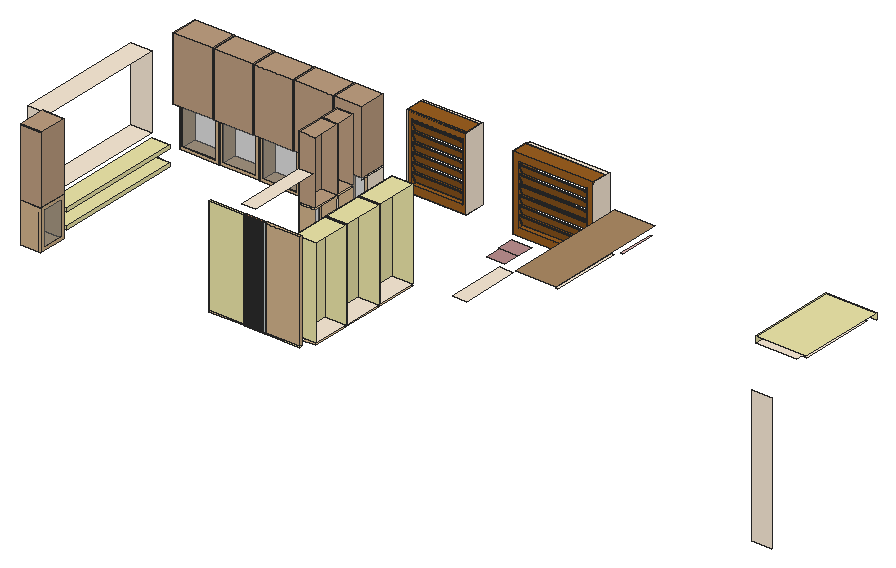
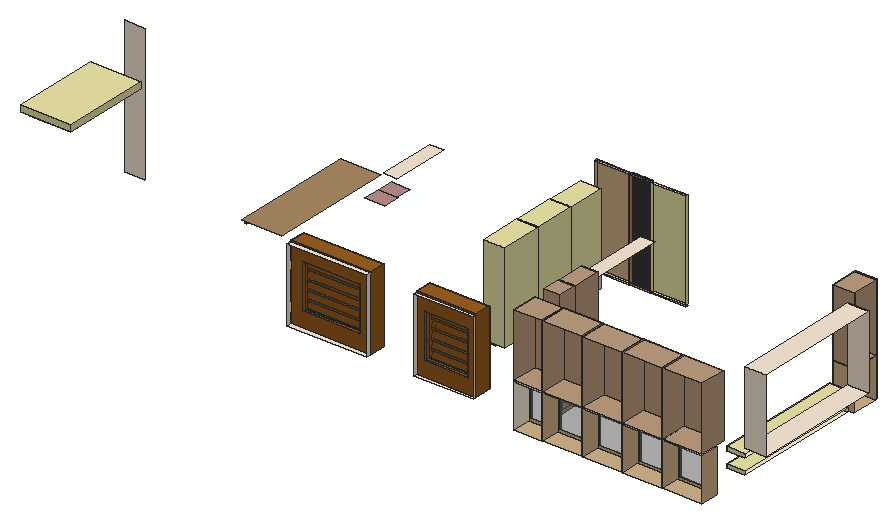
# SketchUp Ruby script. Lengths in inches.
U = 1.inch
M = Sketchup.active_model
def pt(a) = Geom::Point3d.new(a.map { |v| v * U })
def face(e, loops, mat)
  f = e.add_face(loops[0].map { |a| pt(a) })
  loops[1..].each { |l| e.add_face(l.map { |a| pt(a) }).erase! }
  f.material = f.back_material = mat if mat
  f
end
# faces: each face lists its corners as indices into pts; further lists are holes
def faces(e, pts, list, mat = nil) = list.each { |f| face(e, (f[0].is_a?(Array) ? f : [f]).map { |l| l.map { |i| pts[i] } }, mat) }
# xy, xz, yz: faces in a plane at the given z, y or x. An outline is a flat list of corners, or four numbers for a rectangle; further outlines are holes
def ring(l) = l.size == 4 ? [[l[0], l[1]], [l[2], l[1]], [l[2], l[3]], [l[0], l[3]]] : l.each_slice(2).to_a
def flat(e, list, mat, &to3) = list.each { |f| face(e, (f[0].is_a?(Array) ? f : [f]).map { |l| ring(l).map { |u, v| to3.(u, v) } }, mat) }
def xy(e, z, list, mat = nil) = flat(e, list, mat) { |x, y| [x, y, z] }
def xz(e, y, list, mat = nil) = flat(e, list, mat) { |x, z| [x, y, z] }
def yz(e, x, list, mat = nil) = flat(e, list, mat) { |y, z| [x, y, z] }
def lines(e, pts, list) = list.each { |a, b| e.add_line(pt(pts[a]), pt(pts[b])) }
# prism: a flat outline (further loops are holes) pulled along v
def prism(e, loops, v, mat = nil)
  f = face(e, loops, mat); d = Geom::Vector3d.new(v.map { |x| x * U })
  f.pushpull(f.normal.samedirection?(d) ? d.length : -d.length)
end
def box(e, o, s, mat = nil) = prism(e, [[o, [o[0] + s[0], o[1], o[2]], [o[0] + s[0], o[1] + s[1], o[2]], [o[0], o[1] + s[1], o[2]]]], [0, 0, s[2]], mat)
def at(x, y, z, deg = 0) = Geom::Transformation.translation(pt([x, y, z])) * Geom::Transformation.rotation(ORIGIN, Z_AXIS, deg.degrees)
def axes(o, x, y, z) = Geom::Transformation.new([*x, 0, *y, 0, *z, 0, *pt(o).to_a, 1])
def part(name) = M.definitions.add(name)
# library, detail: a bought-in or finely detailed component or shape, given as its bounding box
def library(name, o, s) = part(name).tap { |d| box(d.entities, o, s) }
def detail(e, o, s) = box(e.add_group.entities, o, s)
def put(e, d, t, mat = nil) = e.add_instance(d, t).tap { |i| i.material = mat if mat }
def group(e, t, mat = nil) = e.add_group.tap { |g| g.transformation = t; g.material = mat if mat }.entities
root = M.entities
M.materials.add("Maquette Wood B01 12cm").color = [172, 139, 100]
M.materials.add("Plywood A 50cm\#1").color = [191, 159, 129]
M.materials.add("Wood EXN").color = [155, 95, 32]
M.materials.add("[0028_AntiqueWhite]").color = [250, 235, 215]
M.materials.add("[0035_Tan]").color = [210, 180, 140]
M.materials.add("[0048_PaleGoldenrod]").color = [238, 232, 170]
M.materials.add("[0119_RosyBrown]").color = [188, 143, 143]
M.materials.add("[Textile Leaves Green]").color = [226, 183, 181]
M.materials.add("[Translucent Glass Gray]").color = [128, 128, 128]
M.materials["[Translucent Glass Gray]"].alpha = 0.5
M.materials.add("[Wallpaper Dog Bone]").color = [213, 224, 224]
M.materials.add("[Wood Veneer 02]").color = [190, 128, 91]
c1 = part("Group\#38")
prism(c1.entities,[[[0,1.97,1.57],[0,0.24,0.19],[0,0.22,0.17],[0,0.2,0.14],[0,0.19,0.11],[0,0.2,0.08],[0,0.2,0.05],[0,0.22,0.02],[0,0.24,0],[0,0.27,-0.02],[0,0.3,-0.03],[0,0.34,-0.03],[0,0.37,-0.02],[0,0.39,0],[0,2.36,1.57]]],[-67.04,0,0])
c2 = part("Wood+Window")
g1 = group(c2.entities,at(47.24,0,19.69),"Wood EXN")
g2 = group(g1,at(-47.24,5.91,0))
xy(g2,-19.69,[[0,-5.91,27.56,0]])
xy(g2,-17.72,[[1.97,-3.9375,25.59,0]])
xy(g2,-15.75,[[3.9375,-5.91,23.62,-4.92],[3.9375,-4.92,23.62,-3.9375]])
xy(g2,-3.9375,[[3.9375,-5.91,23.62,-4.92],[3.9375,-4.92,23.62,-3.9375]])
xy(g2,-1.97,[[1.97,-3.9375,25.59,0]])
xy(g2,0,[[0,-5.91,27.56,0]])
xz(g2,-5.91,[[[0,-19.69,27.56,0],[3.9375,-15.75,23.62,-3.9375]]])
xz(g2,-3.9375,[[[1.97,-17.72,25.59,-1.97],[3.9375,-15.75,23.62,-3.9375]]])
xz(g2,0,[[[0,-19.69,27.56,0],[1.97,-17.72,25.59,-1.97]]])
yz(g2,0,[[-5.91,-19.69,0,0]])
yz(g2,1.97,[[-3.9375,-17.72,0,-1.97]])
yz(g2,3.9375,[[-5.91,-15.75,-4.92,-3.9375],[-4.92,-15.75,-3.9375,-3.9375]])
yz(g2,23.62,[[-5.91,-15.75,-4.92,-3.9375],[-4.92,-15.75,-3.9375,-3.9375]])
yz(g2,25.59,[[-3.9375,-17.72,0,-1.97]])
yz(g2,27.56,[[-5.91,-19.69,0,0]])
g3 = group(g1,at(-20.98,5.88,-0.4))
put(g3,c1,axes([-24.3,0,-14.09],[-0.35238,0,0],[0,0,-1.2344],[0,-1,0]))
put(g3,c1,axes([-24.3,0,-11.66],[-0.35238,0,0],[0,0,-1.2344],[0,-1,0]))
put(g3,c1,axes([-24.3,0,-9.23],[-0.35238,0,0],[0,0,-1.2344],[0,-1,0]))
put(g3,c1,axes([-24.3,0,-6.8],[-0.35238,0,0],[0,0,-1.2344],[0,-1,0]))
put(g3,c1,axes([-24.3,0,-4.375],[-0.35238,0,0],[0,0,-1.2344],[0,-1,0]))
put(g3,c1,axes([-24.3,0,-1.94],[-0.35238,0,0],[0,0,-1.2344],[0,-1,0]))
xy(root,67.4375,[[9,365.9375,18.125,377.9375],[86.0625,421,93,433],[86.0625,433.5,93,441.5625],[10,450.9375,27,459],[27.5,450.9375,44.5,459],
  [45,450.9375,62,459],[62.5,450.9375,79.5,459],[80,450.9375,92,459]],"[0035_Tan]")
xy(root,68.47,[[46.04,450.9375,60.96,451.3125]],"[Translucent Glass Gray]")
xy(root,68.57,[[11.13,450.9375,25.87,451.25]],"[Translucent Glass Gray]")
xy(root,68.6,[[17.9375,367.1,18.125,376.78],[28.66,450.9375,43.34,451.25]],"[Translucent Glass Gray]")
xy(root,68.625,[[86.0625,422.1875,86.4375,431.8125]],"[Translucent Glass Gray]")
xy(root,68.67,[[86.0625,434.73,86.25,440.33]],"[Translucent Glass Gray]")
xy(root,68.6875,[[81.25,450.9375,90.75,451.1875]],"[Translucent Glass Gray]")
xy(root,68.7,[[63.76,450.9375,78.24,451.125]],"[Translucent Glass Gray]")
xy(root,69.2,[[9,380.875,16.9375,437.125]],"[0028_AntiqueWhite]")
xy(root,70.71,[[129.3125,369,134.6875,385.5],[129.3125,386,134.6875,403.5],[129.3125,404,134.6875,422]],"[0035_Tan]")
xy(root,70.77,[[9,380.875,16.9375,437.125]],"[0048_PaleGoldenrod]")
xy(root,71.3125,[[125.5625,369.5,134.6875,385.5],[125.5625,386,134.6875,403.5],[125.5625,404,134.6875,422]],"[0028_AntiqueWhite]")
xy(root,72.59,[[94,361.9375,109,363]],"[0035_Tan]")
xy(root,72.59,[[118.6875,361.9375,133.6875,363]],"[0048_PaleGoldenrod]")
xy(root,72.59,[[109.5,361.9375,118.1875,363]],"[Wood Veneer 02]")
xy(root,73.1875,[[109.5,361.5625,109.82,361.9375],[110.02,361.5625,110.35,361.9375],[110.55,361.5625,110.87,361.9375],[111.07,361.5625,111.39,361.9375],[111.59,361.5625,111.92,361.9375],
  [112.12,361.5625,112.44,361.9375],[112.64,361.5625,112.96,361.9375],[113.16,361.5625,113.49,361.9375],[113.6875,361.5625,114.01,361.9375],[114.21,361.5625,114.54,361.9375],
  [114.73,361.5625,115.06,361.9375],[115.26,361.5625,115.58,361.9375],[115.78,361.5625,116.11,361.9375],[116.3,361.5625,116.63,361.9375],[116.83,361.5625,117.15,361.9375],
  [117.35,361.5625,117.68,361.9375],[117.875,361.5625,118.2,361.9375],[109.5,361.9375,118.1875,363]],"[0028_AntiqueWhite]")
xy(root,73.1875,[[118.6875,361.9375,133.6875,363]],"[0035_Tan]")
xy(root,73.1875,[[94,361.9375,109,363]],"[0048_PaleGoldenrod]")
xy(root,76.0625,[[9,380.875,16.9375,437.125]],"[0028_AntiqueWhite]")
xy(root,77.6875,[[9,380.875,16.9375,437.125]],"[0048_PaleGoldenrod]")
xy(root,79.6875,[[0,380.875,9,437.125],[102.5,459,128.4375,468],[148.875,459,183.6875,468]],"[0028_AntiqueWhite]")
xy(root,83.55,[[17.9375,367.1,18.125,376.78]],"[Translucent Glass Gray]")
xy(root,84.71,[[9,365.9375,18.125,377.9375]],"[0035_Tan]")
xy(root,84.86,[[63.76,450.9375,78.24,451.125]],"[Translucent Glass Gray]")
xy(root,84.875,[[81.25,450.9375,90.75,451.1875]],"[Translucent Glass Gray]")
xy(root,84.89,[[86.0625,434.73,86.25,440.33]],"[Translucent Glass Gray]")
xy(root,84.9375,[[86.0625,422.1875,86.4375,431.8125]],"[Translucent Glass Gray]")
xy(root,84.96,[[28.66,450.9375,43.34,451.25]],"[Translucent Glass Gray]")
xy(root,84.99,[[11.13,450.9375,25.87,451.25]],"[Translucent Glass Gray]")
xy(root,85.02,[[9,365.9375,18.125,377.9375]],"Plywood A 50cm\#1")
xy(root,85.09,[[46.04,450.9375,60.96,451.3125]],"[Translucent Glass Gray]")
xy(root,86.125,[[86.0625,421,93,433],[86.0625,433.5,93,441.5625],[10,450.9375,27,459],[27.5,450.9375,44.5,459],[45,450.9375,62,459],
  [62.5,450.9375,79.5,459],[80,450.9375,92,459]],"[0035_Tan]")
xy(root,86.6875,[[86.0625,421,93,433],[86.0625,433.5,93,441.5625],[10,447.5,27,459],[27.5,447.5,44.5,459],[45,447.5,62,459],
  [62.5,447.5,79.5,459],[80,447.5,92,459]],"Plywood A 50cm\#1")
xy(root,103.4,[[212.3125,438.47,213,454.22]],"[Textile Leaves Green]")
xy(root,104.55,[[211.3125,404.13,212.3125,434.43]],"[0028_AntiqueWhite]")
xy(root,106,[[195,402.6875,212.3125,456.8125]],"Maquette Wood B01 12cm")
xy(root,106,[[189,375.81,195,401.3125],[93,381.06,99,412.0625]],"[0028_AntiqueWhite]")
xy(root,106,[[181,404.5,189,411.4375],[180.4375,411.4375,189,418.8125]],"[0119_RosyBrown]")
xy(root,108.8,[[293.125,410.9375,293.125,449.0625,311,449.0625,311,446.36,313.125,446.36,313.125,413.64,311,413.64,311,410.9375]],"[0028_AntiqueWhite]")
xy(root,110.4375,[[125.5625,369.5,134.6875,385.5],[125.5625,386,134.6875,403.5],[125.5625,404,134.6875,422]],"[0048_PaleGoldenrod]")
xy(root,111.5,[[293.125,410.9375,315,449.0625]],"[0048_PaleGoldenrod]")
xy(root,111.66,[[0,380.875,9,437.125],[102.5,459,128.4375,468],[148.875,459,183.6875,468]],"[0028_AntiqueWhite]")
xy(root,114.3125,[[9,365.9375,18.125,377.9375],[86.0625,421,93,433],[86.0625,433.5,93,441.5625],[10,447.5,27,459],[27.5,447.5,44.5,459],
  [45,447.5,62,459],[62.5,447.5,79.5,459],[80,447.5,92,459]],"Plywood A 50cm\#1")
xy(root,115.7,[[118.6875,361.9375,133.6875,363]],"[0035_Tan]")
xy(root,115.7,[[94,361.9375,109,363]],"[0048_PaleGoldenrod]")
xy(root,115.7,[[109.5,361.5625,109.82,361.9375],[110.02,361.5625,110.35,361.9375],[110.55,361.5625,110.87,361.9375],[111.07,361.5625,111.39,361.9375],[111.59,361.5625,111.92,361.9375],
  [112.12,361.5625,112.44,361.9375],[112.64,361.5625,112.96,361.9375],[113.16,361.5625,113.49,361.9375],[113.6875,361.5625,114.01,361.9375],[114.21,361.5625,114.54,361.9375],
  [114.73,361.5625,115.06,361.9375],[115.26,361.5625,115.58,361.9375],[115.78,361.5625,116.11,361.9375],[116.3,361.5625,116.63,361.9375],[116.83,361.5625,117.15,361.9375],
  [117.35,361.5625,117.68,361.9375],[117.875,361.5625,118.2,361.9375]],"[Wallpaper Dog Bone]")
xy(root,115.7,[[109.5,361.9375,118.1875,363]],"[Wood Veneer 02]")
xz(root,361.9375,[[109.5,73.1875,109.82,115.7],[110.02,73.1875,110.35,115.7],[110.55,73.1875,110.87,115.7],[111.07,73.1875,111.39,115.7],[111.59,73.1875,111.92,115.7],
  [112.12,73.1875,112.44,115.7],[112.64,73.1875,112.96,115.7],[113.16,73.1875,113.49,115.7],[113.6875,73.1875,114.01,115.7],[114.21,73.1875,114.54,115.7],
  [114.73,73.1875,115.06,115.7],[115.26,73.1875,115.58,115.7],[115.78,73.1875,116.11,115.7],[116.3,73.1875,116.63,115.7],[116.83,73.1875,117.15,115.7],
  [117.35,73.1875,117.68,115.7],[117.875,73.1875,118.1875,115.7]],"[0028_AntiqueWhite]")
xz(root,361.9375,[[118.6875,73.1875,133.6875,115.7]],"[0035_Tan]")
xz(root,361.9375,[[94,73.1875,109,115.7]],"[0048_PaleGoldenrod]")
xz(root,361.9375,[[109.82,73.1875,110.02,115.7],[110.35,73.1875,110.55,115.7],[110.87,73.1875,111.07,115.7],[111.39,73.1875,111.59,115.7],[111.92,73.1875,112.12,115.7],
  [112.44,73.1875,112.64,115.7],[112.96,73.1875,113.16,115.7],[113.49,73.1875,113.6875,115.7],[114.01,73.1875,114.21,115.7],[114.54,73.1875,114.73,115.7],
  [115.06,73.1875,115.26,115.7],[115.58,73.1875,115.78,115.7],[116.11,73.1875,116.3,115.7],[116.63,73.1875,116.83,115.7],[117.15,73.1875,117.35,115.7],
  [117.68,73.1875,117.875,115.7]],"[Wood Veneer 02]")
xz(root,364.16,[[17.9375,68.72,18.125,83.43]],"[Translucent Glass Gray]")
xz(root,365.4375,[[9,85.02,18.125,114.3125]],"Plywood A 50cm\#1")
xz(root,365.4375,[[9,67.4375,18.125,84.71]],"[0035_Tan]")
xz(root,365.9375,[[9,85.02,18.125,114.3125]],"Plywood A 50cm\#1")
xz(root,365.9375,[[9,67.4375,18.125,84.71]],"[0035_Tan]")
xz(root,367.1,[[17.9375,68.6,18.125,83.55]],"[0028_AntiqueWhite]")
xz(root,369.5,[[125.5625,71.3125,134.6875,110.4375]],"[0048_PaleGoldenrod]")
xz(root,376.78,[[17.9375,68.6,18.125,83.55]],"[0028_AntiqueWhite]")
xz(root,377.9375,[[9,85.02,18.125,114.3125]],"Plywood A 50cm\#1")
xz(root,377.9375,[[9,67.4375,18.125,84.71]],"[0035_Tan]")
xz(root,380.875,[[0,79.6875,9,111.66]],"[0028_AntiqueWhite]")
xz(root,380.875,[[9,69.2,16.9375,70.77],[9,76.0625,16.9375,77.6875]],"[0048_PaleGoldenrod]")
xz(root,381.0625,[[315,52.5,324,111.5]],"[0028_AntiqueWhite]")
xz(root,385.5,[[125.5625,71.3125,134.6875,110.4375]],"[0048_PaleGoldenrod]")
xz(root,386,[[125.5625,71.3125,134.6875,110.4375]],"[0048_PaleGoldenrod]")
xz(root,403.5,[[125.5625,71.3125,134.6875,110.4375]],"[0048_PaleGoldenrod]")
xz(root,404,[[125.5625,71.3125,134.6875,110.4375]],"[0048_PaleGoldenrod]")
xz(root,421,[[86.0625,86.6875,93,114.3125]],"Plywood A 50cm\#1")
xz(root,421,[[86.0625,67.4375,93,86.125]],"[0035_Tan]")
xz(root,422,[[125.5625,71.3125,134.6875,110.4375]],"[0048_PaleGoldenrod]")
xz(root,422.1875,[[86.0625,68.625,86.4375,84.9375]],"[Translucent Glass Gray]")
xz(root,431.8125,[[86.0625,68.625,86.4375,84.9375]],"[Translucent Glass Gray]")
xz(root,433,[[86.0625,86.6875,93,114.3125]],"Plywood A 50cm\#1")
xz(root,433,[[86.0625,67.4375,93,86.125]],"[0035_Tan]")
xz(root,433.5,[[86.0625,86.6875,93,114.3125]],"Plywood A 50cm\#1")
xz(root,433.5,[[86.0625,67.4375,93,86.125]],"[0035_Tan]")
xz(root,434.73,[[86.0625,68.67,86.25,84.89]],"[Translucent Glass Gray]")
xz(root,437.125,[[0,79.6875,9,111.66]],"[0028_AntiqueWhite]")
xz(root,437.125,[[9,69.2,16.9375,70.77],[9,76.0625,16.9375,77.6875]],"[0048_PaleGoldenrod]")
xz(root,440.33,[[86.0625,68.67,86.25,84.89]],"[Translucent Glass Gray]")
xz(root,441.5625,[[86.0625,86.6875,93,114.3125]],"Plywood A 50cm\#1")
xz(root,441.5625,[[86.0625,67.4375,93,86.125]],"[0035_Tan]")
xz(root,447.5,[[10,86.6875,27,114.3125],[27.5,86.6875,44.5,114.3125],[45,86.6875,62,114.3125],[62.5,86.6875,79.5,114.3125],[80,86.6875,92,114.3125]],"Plywood A 50cm\#1")
xz(root,449.0625,[[293.125,108.8,315,111.5]],"[0048_PaleGoldenrod]")
xz(root,450.9375,[[[10,67.4375,27,86.125],[11.13,68.57,25.87,84.99]],[[27.5,67.4375,44.5,86.125],[28.66,68.6,43.34,84.96]],[[45,67.4375,62,86.125],[46.04,68.47,60.96,85.09]],[[62.5,67.4375,79.5,86.125],[63.76,68.7,78.24,84.86]],[[80,67.4375,92,86.125],[81.25,68.6875,90.75,84.875]]],"[0035_Tan]")
xz(root,451.125,[[63.76,68.7,78.24,84.86]],"[Translucent Glass Gray]")
xz(root,451.1875,[[81.25,68.6875,90.75,84.875]],"[Translucent Glass Gray]")
xz(root,451.25,[[11.13,68.57,25.87,84.99],[28.66,68.6,43.34,84.96]],"[Translucent Glass Gray]")
xz(root,451.3125,[[46.04,68.47,60.96,85.09]],"[Translucent Glass Gray]")
xz(root,459,[[27,67.4375,27.5,84.6875],[44.5,67.4375,45,84.6875],[62,67.4375,62.5,84.6875],[79.5,67.4375,80,84.6875]],"[0028_AntiqueWhite]")
yz(root,10,[[447.5,86.6875,459,114.3125]],"Plywood A 50cm\#1")
yz(root,10,[[450.9375,67.4375,459,86.125]],"[0035_Tan]")
yz(root,11.13,[[450.9375,68.57,451.25,84.99]],"[Translucent Glass Gray]")
yz(root,16.9375,[[380.875,69.2,437.125,70.77],[380.875,76.0625,437.125,77.6875]],"[0048_PaleGoldenrod]")
yz(root,17.9375,[[367.1,68.6,376.78,83.55]],"[Translucent Glass Gray]")
yz(root,18.125,[[365.9375,85.02,377.9375,114.3125]],"Plywood A 50cm\#1")
yz(root,18.125,[[[365.9375,67.4375,377.9375,84.71],[367.1,68.6,376.78,83.55]]],"[0035_Tan]")
yz(root,25.87,[[450.9375,68.57,451.25,84.99]],"[Translucent Glass Gray]")
yz(root,27,[[447.5,86.6875,459,114.3125]],"Plywood A 50cm\#1")
yz(root,27,[[450.9375,67.4375,459,86.125]],"[0035_Tan]")
yz(root,27.5,[[447.5,86.6875,459,114.3125]],"Plywood A 50cm\#1")
yz(root,27.5,[[450.9375,67.4375,459,86.125]],"[0035_Tan]")
yz(root,28.66,[[450.9375,68.6,451.25,84.96]],"[Translucent Glass Gray]")
yz(root,43.34,[[450.9375,68.6,451.25,84.96]],"[Translucent Glass Gray]")
yz(root,44.5,[[447.5,86.6875,459,114.3125]],"Plywood A 50cm\#1")
yz(root,44.5,[[450.9375,67.4375,459,86.125]],"[0035_Tan]")
yz(root,45,[[447.5,86.6875,459,114.3125]],"Plywood A 50cm\#1")
yz(root,45,[[450.9375,67.4375,459,86.125]],"[0035_Tan]")
yz(root,46.04,[[450.9375,68.47,451.3125,85.09]],"[Translucent Glass Gray]")
yz(root,60.96,[[450.9375,68.47,451.3125,85.09]],"[Translucent Glass Gray]")
yz(root,62,[[447.5,86.6875,459,114.3125]],"Plywood A 50cm\#1")
yz(root,62,[[450.9375,67.4375,459,86.125]],"[0035_Tan]")
yz(root,62.5,[[447.5,86.6875,459,114.3125]],"Plywood A 50cm\#1")
yz(root,62.5,[[450.9375,67.4375,459,86.125]],"[0035_Tan]")
yz(root,63.76,[[450.9375,68.7,451.125,84.86]],"[Translucent Glass Gray]")
yz(root,78.24,[[450.9375,68.7,451.125,84.86]],"[Translucent Glass Gray]")
yz(root,79.5,[[447.5,86.6875,459,114.3125]],"Plywood A 50cm\#1")
yz(root,79.5,[[450.9375,67.4375,459,86.125]],"[0035_Tan]")
yz(root,80,[[447.5,86.6875,459,114.3125]],"Plywood A 50cm\#1")
yz(root,80,[[450.9375,67.4375,459,86.125]],"[0035_Tan]")
yz(root,81.25,[[450.9375,68.6875,451.1875,84.875]],"[Translucent Glass Gray]")
yz(root,86.0625,[[421,86.6875,433,114.3125],[433.5,86.6875,441.5625,114.3125]],"Plywood A 50cm\#1")
yz(root,86.0625,[[[421,67.4375,433,86.125],[422.1875,68.625,431.8125,84.9375]],[[433.5,67.4375,441.5625,86.125],[434.73,68.67,440.33,84.89]]],"[0035_Tan]")
yz(root,86.25,[[434.73,68.67,440.33,84.89]],"[Translucent Glass Gray]")
yz(root,86.4375,[[422.1875,68.625,431.8125,84.9375]],"[Translucent Glass Gray]")
yz(root,90.75,[[450.9375,68.6875,451.1875,84.875]],"[Translucent Glass Gray]")
yz(root,92,[[447.5,86.6875,459,114.3125]],"Plywood A 50cm\#1")
yz(root,92,[[450.9375,67.4375,459,86.125]],"[0028_AntiqueWhite]")
yz(root,93,[[433,67.4375,433.5,84.6875]],"[0028_AntiqueWhite]")
yz(root,94,[[361.9375,73.1875,363,115.7]],"[0048_PaleGoldenrod]")
yz(root,102.5,[[459,79.6875,468,111.66]],"[0028_AntiqueWhite]")
yz(root,109,[[361.9375,73.1875,363,115.7]],"[0048_PaleGoldenrod]")
yz(root,109.5,[[361.9375,73.1875,363,115.7]],"[Wood Veneer 02]")
yz(root,109.82,[[361.5625,73.1875,361.9375,115.7]],"[Wallpaper Dog Bone]")
yz(root,110.02,[[361.5625,73.1875,361.9375,115.7]],"[Wallpaper Dog Bone]")
yz(root,110.35,[[361.5625,73.1875,361.9375,115.7]],"[Wallpaper Dog Bone]")
yz(root,110.55,[[361.5625,73.1875,361.9375,115.7]],"[Wallpaper Dog Bone]")
yz(root,110.87,[[361.5625,73.1875,361.9375,115.7]],"[Wallpaper Dog Bone]")
yz(root,111.07,[[361.5625,73.1875,361.9375,115.7]],"[Wallpaper Dog Bone]")
yz(root,111.39,[[361.5625,73.1875,361.9375,115.7]],"[Wallpaper Dog Bone]")
yz(root,111.59,[[361.5625,73.1875,361.9375,115.7]],"[Wallpaper Dog Bone]")
yz(root,111.92,[[361.5625,73.1875,361.9375,115.7]],"[Wallpaper Dog Bone]")
yz(root,112.12,[[361.5625,73.1875,361.9375,115.7]],"[Wallpaper Dog Bone]")
yz(root,112.44,[[361.5625,73.1875,361.9375,115.7]],"[Wallpaper Dog Bone]")
yz(root,112.64,[[361.5625,73.1875,361.9375,115.7]],"[Wallpaper Dog Bone]")
yz(root,112.96,[[361.5625,73.1875,361.9375,115.7]],"[Wallpaper Dog Bone]")
yz(root,113.16,[[361.5625,73.1875,361.9375,115.7]],"[Wallpaper Dog Bone]")
yz(root,113.49,[[361.5625,73.1875,361.9375,115.7]],"[Wallpaper Dog Bone]")
yz(root,113.6875,[[361.5625,73.1875,361.9375,115.7]],"[Wallpaper Dog Bone]")
yz(root,114.01,[[361.5625,73.1875,361.9375,115.7]],"[Wallpaper Dog Bone]")
yz(root,114.21,[[361.5625,73.1875,361.9375,115.7]],"[Wallpaper Dog Bone]")
yz(root,114.54,[[361.5625,73.1875,361.9375,115.7]],"[Wallpaper Dog Bone]")
yz(root,114.73,[[361.5625,73.1875,361.9375,115.7]],"[Wallpaper Dog Bone]")
yz(root,115.06,[[361.5625,73.1875,361.9375,115.7]],"[Wallpaper Dog Bone]")
yz(root,115.26,[[361.5625,73.1875,361.9375,115.7]],"[Wallpaper Dog Bone]")
yz(root,115.58,[[361.5625,73.1875,361.9375,115.7]],"[Wallpaper Dog Bone]")
yz(root,115.78,[[361.5625,73.1875,361.9375,115.7]],"[Wallpaper Dog Bone]")
yz(root,116.11,[[361.5625,73.1875,361.9375,115.7]],"[Wallpaper Dog Bone]")
yz(root,116.3,[[361.5625,73.1875,361.9375,115.7]],"[Wallpaper Dog Bone]")
yz(root,116.63,[[361.5625,73.1875,361.9375,115.7]],"[Wallpaper Dog Bone]")
yz(root,116.83,[[361.5625,73.1875,361.9375,115.7]],"[Wallpaper Dog Bone]")
yz(root,117.15,[[361.5625,73.1875,361.9375,115.7]],"[Wallpaper Dog Bone]")
yz(root,117.35,[[361.5625,73.1875,361.9375,115.7]],"[Wallpaper Dog Bone]")
yz(root,117.68,[[361.5625,73.1875,361.9375,115.7]],"[Wallpaper Dog Bone]")
yz(root,117.875,[[361.5625,73.1875,361.9375,115.7]],"[Wallpaper Dog Bone]")
yz(root,118.1875,[[361.9375,73.1875,363,115.7]],"[Wood Veneer 02]")
yz(root,118.2,[[361.5625,73.1875,361.9375,115.7]],"[Wallpaper Dog Bone]")
yz(root,118.6875,[[361.9375,73.1875,363,115.7]],"[0035_Tan]")
yz(root,125.5625,[[369.5,71.3125,385.5,110.4375],[386,71.3125,403.5,110.4375],[404,71.3125,422,110.4375]],"[0048_PaleGoldenrod]")
yz(root,128.4375,[[459,79.6875,468,111.66]],"[0028_AntiqueWhite]")
yz(root,133.6875,[[361.9375,73.1875,363,115.7]],"[0035_Tan]")
yz(root,148.875,[[459,79.6875,468,111.66]],"[0028_AntiqueWhite]")
yz(root,183.6875,[[459,79.6875,468,111.66]],"[0028_AntiqueWhite]")
yz(root,293.125,[[410.9375,108.8,449.0625,111.5]],"[0048_PaleGoldenrod]")
p = [[93,458,86.6875],[93,446,86.6875],[93,458,67.4375],[93,458,84.6875]]
lines(root,p,[[0,1],[2,3]])
put(root,c2,axes([183.6875,465.72,79.6875],[-1.2632,0,0],[0,-1.15534,0],[0,0,1.6463]))
put(root,c2,axes([128.4375,466.61,79.6875],[-0.94116,0,0],[0,-1.22958,0],[0,0,1.6463]))
